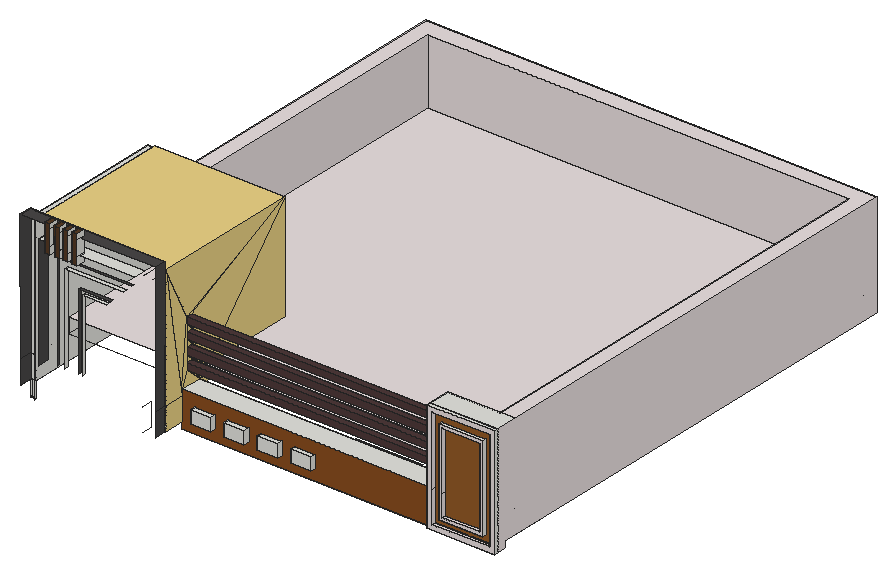
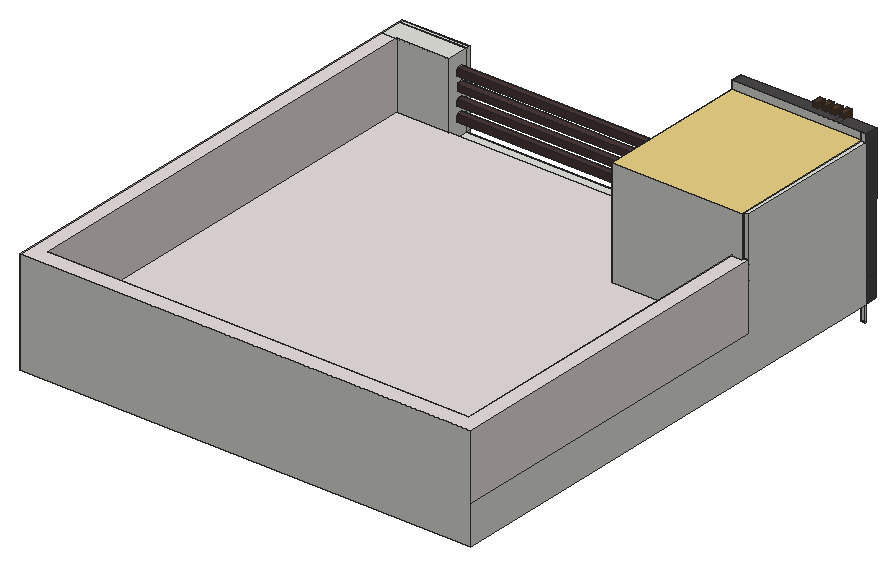
# SketchUp Ruby script. Lengths in inches.
U = 1.inch
M = Sketchup.active_model
def pt(a) = Geom::Point3d.new(a.map { |v| v * U })
def face(e, loops, mat)
  f = e.add_face(loops[0].map { |a| pt(a) })
  loops[1..].each { |l| e.add_face(l.map { |a| pt(a) }).erase! }
  f.material = f.back_material = mat if mat
  f
end
# faces: each face lists its corners as indices into pts; further lists are holes
def faces(e, pts, list, mat = nil) = list.each { |f| face(e, (f[0].is_a?(Array) ? f : [f]).map { |l| l.map { |i| pts[i] } }, mat) }
# xy, xz, yz: faces in a plane at the given z, y or x. An outline is a flat list of corners, or four numbers for a rectangle; further outlines are holes
def ring(l) = l.size == 4 ? [[l[0], l[1]], [l[2], l[1]], [l[2], l[3]], [l[0], l[3]]] : l.each_slice(2).to_a
def flat(e, list, mat, &to3) = list.each { |f| face(e, (f[0].is_a?(Array) ? f : [f]).map { |l| ring(l).map { |u, v| to3.(u, v) } }, mat) }
def xy(e, z, list, mat = nil) = flat(e, list, mat) { |x, y| [x, y, z] }
def xz(e, y, list, mat = nil) = flat(e, list, mat) { |x, z| [x, y, z] }
def yz(e, x, list, mat = nil) = flat(e, list, mat) { |y, z| [x, y, z] }
def lines(e, pts, list) = list.each { |a, b| e.add_line(pt(pts[a]), pt(pts[b])) }
# prism: a flat outline (further loops are holes) pulled along v
def prism(e, loops, v, mat = nil)
  f = face(e, loops, mat); d = Geom::Vector3d.new(v.map { |x| x * U })
  f.pushpull(f.normal.samedirection?(d) ? d.length : -d.length)
end
def box(e, o, s, mat = nil) = prism(e, [[o, [o[0] + s[0], o[1], o[2]], [o[0] + s[0], o[1] + s[1], o[2]], [o[0], o[1] + s[1], o[2]]]], [0, 0, s[2]], mat)
def at(x, y, z, deg = 0) = Geom::Transformation.translation(pt([x, y, z])) * Geom::Transformation.rotation(ORIGIN, Z_AXIS, deg.degrees)
def axes(o, x, y, z) = Geom::Transformation.new([*x, 0, *y, 0, *z, 0, *pt(o).to_a, 1])
def part(name) = M.definitions.add(name)
# library, detail: a bought-in or finely detailed component or shape, given as its bounding box
def library(name, o, s) = part(name).tap { |d| box(d.entities, o, s) }
def detail(e, o, s) = box(e.add_group.entities, o, s)
def put(e, d, t, mat = nil) = e.add_instance(d, t).tap { |i| i.material = mat if mat }
def group(e, t, mat = nil) = e.add_group.tap { |g| g.transformation = t; g.material = mat if mat }.entities
root = M.entities
M.materials.add("Generic").color = [136, 77, 32]
M.materials.add("Generic\#1").color = [73, 71, 71]
M.materials.add("Generic\#2").color = [78, 57, 57]
M.materials.add("Generic\#3").color = [235, 210, 133]
M.materials.add("Generic\#4").color = [84, 58, 36]
M.materials.add("Generic\#5").color = [232, 222, 222]
M.materials.add("Material \#1").color = [140, 140, 140]
M.materials.add("[Wood Floor Parquet]").color = [145, 89, 39]
xy(root,225.757,[[371.53,115.15,371.464,115.17,371.474,115.185],[371.53,115.15,371.474,115.185,371.533,115.167],[371.53,115.15,371.533,115.167,371.6,115.15],[371.6,115.15,371.533,115.167,371.597,115.167],[371.6,115.15,371.597,115.167,371.667,115.17],
  [371.597,115.167,371.657,115.185,371.667,115.17],[371.464,115.17,371.41,115.209,371.425,115.22],[371.464,115.17,371.425,115.22,371.474,115.185],[371.667,115.17,371.657,115.185,371.721,115.209],[371.657,115.185,371.705,115.22,371.721,115.209],
  [371.41,115.209,371.374,115.261,371.393,115.267],[371.41,115.209,371.393,115.267,371.425,115.22],[371.721,115.209,371.705,115.22,371.756,115.261],[371.705,115.22,371.737,115.267,371.756,115.261],[371.374,115.261,371.362,115.32,371.382,115.32],
  [371.374,115.261,371.382,115.32,371.393,115.267],[371.756,115.261,371.737,115.267,371.768,115.32],[371.737,115.267,371.748,115.32,371.768,115.32],[371.362,115.32,371.374,115.379,371.393,115.373],[371.362,115.32,371.393,115.373,371.382,115.32],
  [371.748,115.32,371.737,115.373,371.756,115.379],[371.748,115.32,371.756,115.379,371.768,115.32],[371.393,115.373,371.374,115.379,371.425,115.42],[371.737,115.373,371.705,115.42,371.721,115.431],[371.737,115.373,371.721,115.431,371.756,115.379],
  [371.374,115.379,371.41,115.431,371.425,115.42],[371.425,115.42,371.41,115.431,371.474,115.454],[371.705,115.42,371.657,115.454,371.667,115.469],[371.705,115.42,371.667,115.469,371.721,115.431],[371.41,115.431,371.464,115.469,371.474,115.454],
  [371.474,115.454,371.464,115.469,371.533,115.473],[371.657,115.454,371.597,115.473,371.6,115.49],[371.657,115.454,371.6,115.49,371.667,115.469],[371.464,115.469,371.53,115.49,371.533,115.473],[371.533,115.473,371.53,115.49,371.597,115.473],
  [371.597,115.473,371.53,115.49,371.6,115.49]],"Material \#1")
xy(root,225.773,[[371.53,115.15,371.533,115.167,371.464,115.17],[371.53,115.15,371.597,115.167,371.533,115.167],[371.53,115.15,371.6,115.15,371.597,115.167],[371.6,115.15,371.657,115.185,371.597,115.167],[371.6,115.15,371.667,115.17,371.657,115.185],
  [371.533,115.167,371.474,115.185,371.464,115.17],[371.464,115.17,371.474,115.185,371.41,115.209],[371.667,115.17,371.705,115.22,371.657,115.185],[371.667,115.17,371.721,115.209,371.705,115.22],[371.474,115.185,371.425,115.22,371.41,115.209],
  [371.41,115.209,371.425,115.22,371.374,115.261],[371.721,115.209,371.737,115.267,371.705,115.22],[371.721,115.209,371.756,115.261,371.737,115.267],[371.425,115.22,371.393,115.267,371.374,115.261],[371.374,115.261,371.393,115.267,371.362,115.32],
  [371.756,115.261,371.748,115.32,371.737,115.267],[371.756,115.261,371.768,115.32,371.748,115.32],[371.393,115.267,371.382,115.32,371.362,115.32],[371.362,115.32,371.382,115.32,371.374,115.379],[371.382,115.32,371.393,115.373,371.374,115.379],
  [371.748,115.32,371.768,115.32,371.737,115.373],[371.768,115.32,371.756,115.379,371.737,115.373],[371.393,115.373,371.41,115.431,371.374,115.379],[371.393,115.373,371.425,115.42,371.41,115.431],[371.737,115.373,371.756,115.379,371.705,115.42],
  [371.756,115.379,371.721,115.431,371.705,115.42],[371.425,115.42,371.464,115.469,371.41,115.431],[371.425,115.42,371.474,115.454,371.464,115.469],[371.705,115.42,371.721,115.431,371.657,115.454],[371.721,115.431,371.667,115.469,371.657,115.454],
  [371.474,115.454,371.53,115.49,371.464,115.469],[371.474,115.454,371.533,115.473,371.53,115.49],[371.657,115.454,371.667,115.469,371.597,115.473],[371.667,115.469,371.6,115.49,371.597,115.473],[371.533,115.473,371.6,115.49,371.53,115.49],
  [371.533,115.473,371.597,115.473,371.6,115.49]],"Material \#1")
xy(root,227.533,[[205.199,114.8125,268.449,169.8125]])
xy(root,229.316,[[371.53,115.15,371.464,115.17,371.533,115.167],[371.53,115.15,371.533,115.167,371.597,115.167],[371.53,115.15,371.597,115.167,371.6,115.15],[371.6,115.15,371.597,115.167,371.657,115.185],[371.6,115.15,371.657,115.185,371.667,115.17],
  [371.533,115.167,371.464,115.17,371.474,115.185],[371.464,115.17,371.41,115.209,371.474,115.185],[371.667,115.17,371.657,115.185,371.705,115.22],[371.667,115.17,371.705,115.22,371.721,115.209],[371.474,115.185,371.41,115.209,371.425,115.22],
  [371.41,115.209,371.374,115.261,371.425,115.22],[371.721,115.209,371.705,115.22,371.737,115.267],[371.721,115.209,371.737,115.267,371.756,115.261],[371.425,115.22,371.374,115.261,371.393,115.267],[371.374,115.261,371.362,115.32,371.393,115.267],
  [371.756,115.261,371.737,115.267,371.748,115.32],[371.756,115.261,371.748,115.32,371.768,115.32],[371.393,115.267,371.362,115.32,371.382,115.32],[371.362,115.32,371.374,115.379,371.382,115.32],[371.382,115.32,371.374,115.379,371.393,115.373],
  [371.748,115.32,371.737,115.373,371.768,115.32],[371.768,115.32,371.737,115.373,371.756,115.379],[371.393,115.373,371.374,115.379,371.41,115.431],[371.393,115.373,371.41,115.431,371.425,115.42],[371.737,115.373,371.705,115.42,371.756,115.379],
  [371.756,115.379,371.705,115.42,371.721,115.431],[371.425,115.42,371.41,115.431,371.464,115.469],[371.425,115.42,371.464,115.469,371.474,115.454],[371.705,115.42,371.657,115.454,371.721,115.431],[371.721,115.431,371.657,115.454,371.667,115.469],
  [371.474,115.454,371.464,115.469,371.53,115.49],[371.474,115.454,371.53,115.49,371.533,115.473],[371.657,115.454,371.597,115.473,371.667,115.469],[371.667,115.469,371.597,115.473,371.6,115.49],[371.533,115.473,371.53,115.49,371.6,115.49],
  [371.533,115.473,371.6,115.49,371.597,115.473]],"Material \#1")
xy(root,229.332,[[371.53,115.15,371.474,115.185,371.464,115.17],[371.53,115.15,371.533,115.167,371.474,115.185],[371.53,115.15,371.6,115.15,371.533,115.167],[371.6,115.15,371.597,115.167,371.533,115.167],[371.6,115.15,371.667,115.17,371.597,115.167],
  [371.597,115.167,371.667,115.17,371.657,115.185],[371.464,115.17,371.425,115.22,371.41,115.209],[371.464,115.17,371.474,115.185,371.425,115.22],[371.667,115.17,371.721,115.209,371.657,115.185],[371.657,115.185,371.721,115.209,371.705,115.22],
  [371.41,115.209,371.393,115.267,371.374,115.261],[371.41,115.209,371.425,115.22,371.393,115.267],[371.721,115.209,371.756,115.261,371.705,115.22],[371.705,115.22,371.756,115.261,371.737,115.267],[371.374,115.261,371.382,115.32,371.362,115.32],
  [371.374,115.261,371.393,115.267,371.382,115.32],[371.756,115.261,371.768,115.32,371.737,115.267],[371.737,115.267,371.768,115.32,371.748,115.32],[371.362,115.32,371.382,115.32,371.393,115.373],[371.362,115.32,371.393,115.373,371.374,115.379],
  [371.748,115.32,371.756,115.379,371.737,115.373],[371.748,115.32,371.768,115.32,371.756,115.379],[371.393,115.373,371.425,115.42,371.374,115.379],[371.737,115.373,371.721,115.431,371.705,115.42],[371.737,115.373,371.756,115.379,371.721,115.431],
  [371.374,115.379,371.425,115.42,371.41,115.431],[371.425,115.42,371.474,115.454,371.41,115.431],[371.705,115.42,371.667,115.469,371.657,115.454],[371.705,115.42,371.721,115.431,371.667,115.469],[371.41,115.431,371.474,115.454,371.464,115.469],
  [371.474,115.454,371.533,115.473,371.464,115.469],[371.657,115.454,371.6,115.49,371.597,115.473],[371.657,115.454,371.667,115.469,371.6,115.49],[371.464,115.469,371.533,115.473,371.53,115.49],[371.533,115.473,371.597,115.473,371.53,115.49],
  [371.597,115.473,371.6,115.49,371.53,115.49]],"Material \#1")
xy(root,235.716,[[330.35,114.8125,374.475,141.3125]])
xy(root,255.6875,[[361.519,58.125,424.885,61.6875],[127.575,61.6875,402.977,70.125],[402.977,61.6875,412.79,70.125],[412.79,61.6875,419.477,70.125],[419.477,61.6875,424.885,70.125]])
xy(root,260.286,[[366.118,58.125,420.286,61.6875]],"Generic\#5")
xy(root,261.937,[[0.012,30.0625,0.509,42.5]])
xy(root,261.9375,[[4.322,41.4375,4.387,42.5],[4.387,41.4375,4.884,42.5],[4.322,42.5,4.884,42.5,4.885,114.8125,4.322,114.8125],[412.79,70.125,419.477,79.528]])
xy(root,261.9375,[[127.575,70.125,127.575,114.8125,424.885,114.8125,424.885,70.125,419.477,70.125,419.477,79.528,412.79,79.528,412.79,70.125]],"Generic\#3")
xy(root,266.347,[[139.227,56.9375,158.441,61.6875],[170.664,56.9375,189.878,61.6875],[202.102,56.9375,221.316,61.6875],[233.539,56.9375,252.753,61.6875]])
xy(root,266.989,[[372.821,58.125,413.583,61.6875]],"Generic\#5")
xy(root,269.637,[[375.469,58.125,410.935,61.6875]],"Generic\#5")
xy(root,278.222,[[139.227,56.9375,158.441,61.6875],[170.664,56.9375,189.878,61.6875],[202.102,56.9375,221.316,61.6875],[233.539,56.9375,252.753,61.6875]])
xy(root,289.375,[[127.57,61.6875,361.519,82.1875]])
xy(root,298,[[4.322,82.1875,411.072,82.1875,411.072,493.0625,14.375,493.0625,14.375,180.616,4.322,180.616]],"Generic\#5")
xy(root,345.113,[[375.469,58.125,410.935,61.6875]],"Generic\#5")
xy(root,347.761,[[372.821,58.125,413.583,61.6875]])
xy(root,351.982,[[51.311,39.25,73.882,42.5]])
xy(root,355.589,[[366.118,58.125,420.286,61.6875]],"Generic\#5")
xy(root,355.683,[[47.609,39.25,77.584,42.5]],"Generic\#1")
xy(root,360.1875,[[361.519,58.125,424.885,61.6875],[361.519,61.6875,424.885,82.1875]])
xy(root,360.1875,[[411.072,82.1875,424.885,82.1875,424.885,508.6875,0,508.6875,0,180.616,14.375,180.616,14.375,493.0625,411.072,493.0625]],"Generic\#5")
xy(root,368.38,[[34.912,39.25,90.279,42.5]])
xy(root,375.663,[[27.628,39.25,97.5625,41.4375]],"Generic\#1")
xy(root,384.421,[[26.151,26.375,31.026,41.4375],[35.089,26.375,39.964,34.4375],[43.339,26.375,48.214,34.4375],[51.589,26.375,56.464,34.4375]],"Generic\#4")
xy(root,391.47,[[17.071,30.0625,26.151,41.4375],[31.026,30.0625,108.119,41.4375]])
xy(root,398.914,[[0,42.5,4.322,180.616]])
xy(root,406.289,[[0,30.0625,26.108,30.0625,26.108,41.4375,4.322,41.4375,4.322,42.5,0,42.5],[26.108,34.4375,30.983,41.4375]],"Generic\#1")
xy(root,410.825,[[26.095,26.375,30.97,34.4375],[35.033,26.375,39.908,34.4375],[43.283,26.375,48.158,34.4375],[51.533,26.375,56.408,34.4375]],"Generic\#4")
xz(root,26.375,[[26.151,384.421,31.026,384.421,31.026,391.47,30.983,406.289,30.97,410.825,26.095,410.825,26.151,391.47],[35.089,384.421,39.964,384.421,39.964,391.47,39.921,406.289,39.908,410.825,35.033,410.825,35.089,391.47],[43.339,384.421,48.214,384.421,48.214,391.47,48.171,406.289,48.158,410.825,43.283,410.825,43.339,391.47],[51.589,384.421,56.464,384.421,56.464,391.47,56.421,406.289,56.408,410.825,51.533,410.825,51.589,391.47]],"Generic\#4")
xz(root,34.4375,[[35.089,384.421,35.089,391.47,35.033,410.825,39.908,410.825,39.921,406.289,39.964,391.47,39.964,384.421],[43.339,384.421,43.339,391.47,43.283,410.825,48.158,410.825,48.171,406.289,48.214,391.47,48.214,384.421],[51.589,384.421,51.589,391.47,51.533,410.825,56.408,410.825,56.421,406.289,56.464,391.47,56.464,384.421],[26.108,406.289,26.095,410.825,30.97,410.825,30.983,406.289]],"Generic\#4")
xz(root,41.4375,[[26.151,384.421,31.026,391.47],[4.322,398.914,4.375,406.289],[4.375,398.914,4.375,406.289,30.983,406.289,127.563,406.29,127.563,398.915]])
xz(root,42.5,[[0.001,246.511,0.51,247.422],[0.51,246.511,4.885,247.422],[0.001,247.422,0.51,247.422,0.509,261.937,0.012,261.937,0,261.9375],[0.51,247.422,4.885,247.422,4.884,261.9375,3.682,261.9375,0.509,261.937],[0.012,261.937,0.008,283.875,0,398.914,0,261.9375],
  [0.012,261.937,0.509,261.937,3.682,261.9375,4.322,261.9375,4.322,283.875,0.008,283.875],[0.008,283.875,4.322,283.875,4.322,398.914,0,398.914],[0,398.914,4.322,406.289]])
xz(root,56.9375,[[139.227,266.347,158.441,278.222],[170.664,266.347,189.878,278.222],[202.102,266.347,221.316,278.222],[233.539,266.347,252.753,278.222]])
xz(root,58.125,[[[361.519,255.6875,424.885,360.1875],[366.118,260.286,420.286,355.589]],[[372.821,266.989,413.583,347.761],[375.469,269.637,410.935,345.113]]],"Generic\#5")
xz(root,61.6875,[[[361.519,255.6875,424.885,360.1875],[366.118,260.286,420.286,355.589]]])
xz(root,61.6875,[[[127.575,255.6875,361.519,255.6875,361.519,289.375,127.57,289.375,127.57,283.875,127.575,261.9375],[233.539,266.347,252.753,278.222],[202.102,266.347,221.316,278.222],[170.664,266.347,189.878,278.222],[139.227,266.347,158.441,278.222]]],"Generic")
xz(root,61.6875,[[[366.118,260.286,420.286,355.589],[372.821,266.989,413.583,347.761]],[375.469,269.637,410.935,345.113]],"[Wood Floor Parquet]")
xz(root,67,[[361.518,316.263,361.519,316.263,361.519,322.513]])
xz(root,67,[[127.568,303.307,361.519,303.322,361.519,303.5625,361.518,309.572,127.568,309.557],[127.568,316.247,361.518,316.263,361.519,322.513,127.568,322.497],[127.568,329.1875,361.52,329.203,361.519,335.453,127.568,335.4375],[127.568,342.128,361.395,342.143,361.394,348.393,127.568,348.378]],"Generic\#2")
xz(root,70.125,[[127.575,255.6875,402.977,261.9375],[402.977,255.6875,412.79,261.9375],[412.79,255.6875,419.477,261.9375],[419.477,255.6875,424.885,261.9375]])
xz(root,73.25,[[361.518,316.263,361.519,322.513,361.519,316.263]])
xz(root,73.25,[[127.568,303.307,127.568,309.557,361.518,309.572,361.519,303.5625,361.519,303.322],[127.568,316.247,127.568,322.497,361.519,322.513,361.518,316.263],[127.568,329.1875,127.568,335.4375,361.519,335.453,361.52,329.203],[127.568,342.128,127.568,348.378,361.394,348.393,361.395,342.143]],"Generic\#2")
xz(root,81.25,[[116.45,261.937,118.45,261.9375,118.445,283.875,116.445,283.875]])
xz(root,82.1875,[[127.57,283.875,361.519,289.375],[361.519,298,411.072,360.1875]])
xz(root,180.616,[[0,360.1875,4.322,398.914]])
xz(root,180.616,[[0,298,4.322,360.1875],[4.322,298,14.375,360.1875]],"Generic\#5")
xz(root,183.125,[[4.383,283.875,4.375,398.914,127.563,398.915,127.57,283.875]])
xz(root,493.0625,[[14.375,298,411.072,360.1875]],"Generic\#5")
xz(root,508.6875,[[0,261.9375,424.885,360.1875]])
yz(root,0,[[42.5,261.9375,42.5,398.914,180.616,398.914,180.616,298,508.6875,298,508.6875,261.9375]])
yz(root,0,[[180.616,298,508.6875,360.1875]],"Generic\#5")
yz(root,4.322,[[41.4375,261.9375,42.5,283.875],[42.5,261.9375,493.6875,261.9375,493.6875,283.875,82.1875,283.875,82.1875,298,180.616,298,180.616,398.914,42.5,398.914],[41.4375,283.875,42.5,406.289]])
yz(root,4.885,[[41.4375,246.511,42.5,247.422]])
yz(root,14.375,[[180.616,298,493.0625,360.1875]],"Generic\#5")
yz(root,26.151,[[26.375,384.421,41.4375,391.47]],"Generic\#4")
yz(root,31.026,[[26.375,384.421,41.4375,391.47]])
yz(root,35.089,[[26.375,384.421,34.4375,391.47]],"Generic\#4")
yz(root,39.964,[[26.375,384.421,34.4375,391.47]])
yz(root,43.339,[[26.375,384.421,34.4375,391.47]],"Generic\#4")
yz(root,48.214,[[26.375,384.421,34.4375,391.47]])
yz(root,51.589,[[26.375,384.421,34.4375,391.47]],"Generic\#4")
yz(root,56.464,[[26.375,384.421,34.4375,391.47]])
yz(root,127.568,[[67,309.557,73.25,309.557,67,316.247],[73.25,309.557,73.25,316.247,67,316.247],[67,322.497,73.25,322.497,67,329.1875],[73.25,322.497,73.25,329.1875,67,329.1875],[67,335.4375,73.25,335.4375,67,342.128],
  [73.25,335.4375,73.25,342.128,67,342.128]],"Generic\#3")
yz(root,127.57,[[82.1875,283.875,183.125,283.875,82.1875,289.375]],"Generic\#3")
yz(root,139.227,[[56.9375,266.347,61.6875,278.222]])
yz(root,158.441,[[56.9375,266.347,61.6875,278.222]])
yz(root,170.664,[[56.9375,266.347,61.6875,278.222]])
yz(root,189.878,[[56.9375,266.347,61.6875,278.222]])
yz(root,202.102,[[56.9375,266.347,61.6875,278.222]])
yz(root,221.316,[[56.9375,266.347,61.6875,278.222]])
yz(root,233.539,[[56.9375,266.347,61.6875,278.222]])
yz(root,252.753,[[56.9375,266.347,61.6875,278.222]])
yz(root,361.519,[[58.125,255.6875,61.6875,289.375],[58.125,289.375,61.6875,360.1875],[61.6875,289.375,82.1875,360.1875],[67,316.263,73.25,322.513]])
yz(root,366.118,[[58.125,260.286,61.6875,289.375],[58.125,289.375,61.6875,355.589]],"Generic\#5")
yz(root,372.821,[[58.125,289.375,61.6875,347.761]])
yz(root,372.821,[[58.125,266.989,61.6875,289.375]],"Generic\#5")
yz(root,375.469,[[58.125,269.637,61.6875,289.375],[58.125,289.375,61.6875,345.113]],"Generic\#5")
yz(root,410.935,[[58.125,269.637,61.6875,345.113]],"Generic\#5")
yz(root,411.072,[[82.1875,298,493.0625,360.1875]],"Generic\#5")
yz(root,413.583,[[58.125,266.989,61.6875,347.761]])
yz(root,420.286,[[58.125,260.286,61.6875,355.589]],"Generic\#5")
yz(root,424.885,[[58.125,255.6875,61.6875,360.1875]])
yz(root,424.885,[[61.6875,255.6875,70.125,255.6875,70.125,261.9375,508.6875,261.9375,508.6875,360.1875,61.6875,360.1875]],"Generic\#5")
p = [[4.884,42.5,261.9375],[4.885,42.5,247.422],[4.885,41.4375,247.422],[4.884,41.4375,261.9375],[0.008,42.5,283.875],[0.012,42.5,261.937],
  [0.012,30.0625,261.937],[0.008,30.0625,283.875],[127.575,30.0625,261.9375],[127.575,41.4375,261.9375],[127.57,41.4375,283.875],[127.57,30.0625,283.875],
  [127.575,42.5,261.9375],[127.57,42.5,283.875],[127.57,61.6875,283.875],[127.575,61.6875,261.9375],[0,42.5,398.914],[0,30.0625,406.289],
  [0,42.5,406.289],[17.077,30.0625,283.877],[17.077,41.4375,283.877],[17.071,41.4375,391.47],[17.071,30.0625,391.47],[127.563,41.4375,398.915],
  [127.563,41.4375,406.29],[127.563,30.0625,406.29],[27.628,39.25,375.663],[27.628,41.4375,375.663],[27.634,41.4375,283.878],[27.634,39.25,283.878],
  [34.917,42.5,283.879],[34.912,42.5,368.38],[34.912,39.25,368.38],[34.917,39.25,283.879],[47.609,42.5,355.683],[47.614,42.5,283.881],
  [47.614,39.25,283.881],[47.609,39.25,355.683],[51.316,42.5,283.882],[51.311,42.5,351.982],[51.311,39.25,351.982],[51.316,39.25,283.882],
  [127.563,42.5,398.915],[127.57,61.6875,289.375],[127.57,183.125,283.875],[127.563,183.125,398.915],[127.57,82.1875,289.375],[127.568,67,348.378],
  [127.568,67,303.307],[127.568,67,309.557],[127.568,67,316.247],[127.568,67,322.497],[127.568,67,329.1875],[127.568,67,335.4375],
  [127.568,67,342.128],[127.568,73.25,303.307],[127.568,73.25,309.557],[127.568,73.25,316.247],[127.568,73.25,322.497],[127.568,73.25,329.1875],
  [127.568,73.25,335.4375],[127.568,73.25,342.128],[127.568,73.25,348.378],[361.519,73.25,303.322],[361.519,67,303.322],[361.518,67,309.572],
  [361.519,67,303.5625],[361.519,73.25,303.5625],[361.518,73.25,309.572],[361.518,73.25,316.263],[361.519,73.25,316.263],[361.519,67,316.263],
  [361.518,67,316.263],[361.519,67,322.513],[361.519,73.25,322.513],[361.52,73.25,329.203],[361.52,67,329.203],[361.519,67,335.453],
  [361.519,73.25,335.453],[361.395,73.25,342.143],[361.395,67,342.143],[361.394,67,348.393],[361.394,73.25,348.393],[26.151,30.0625,391.47],
  [26.151,26.375,391.47],[26.095,26.375,410.825],[26.095,34.4375,410.825],[26.108,34.4375,406.289],[26.108,30.0625,406.289],[31.026,30.0625,391.47],
  [30.983,30.0625,406.289],[30.983,26.375,406.289],[31.026,26.375,391.47],[35.089,26.375,391.47],[35.033,26.375,410.825],[35.033,34.4375,410.825],
  [35.089,34.4375,391.47],[35.089,30.0625,391.47],[39.921,26.375,406.289],[39.964,26.375,391.47],[39.964,30.0625,391.47],[39.964,34.4375,391.47],
  [39.921,34.4375,406.289],[39.921,30.0625,406.289],[43.339,26.375,391.47],[43.283,26.375,410.825],[43.283,34.4375,410.825],[43.339,34.4375,391.47],
  [43.339,30.0625,391.47],[48.171,26.375,406.289],[48.214,26.375,391.47],[48.214,30.0625,391.47],[48.214,34.4375,391.47],[48.171,34.4375,406.289],
  [48.171,30.0625,406.289],[51.589,26.375,391.47],[51.533,26.375,410.825],[51.533,34.4375,410.825],[51.589,34.4375,391.47],[51.589,30.0625,391.47],
  [56.421,26.375,406.289],[56.464,26.375,391.47],[56.464,30.0625,391.47],[56.464,34.4375,391.47],[56.421,34.4375,406.289],[56.421,30.0625,406.289],
  [4.375,183.125,398.914],[4.375,41.4375,398.914],[30.97,34.4375,410.825],[30.97,26.375,410.825],[30.983,34.4375,406.289],[39.908,26.375,410.825],
  [39.908,34.4375,410.825],[48.158,26.375,410.825],[48.158,34.4375,410.825],[56.408,26.375,410.825],[56.408,34.4375,410.825],[30.983,41.4375,406.289],
  [424.885,493.6875,283.875],[4.322,493.6875,283.875],[4.322,61.6875,283.875],[4.383,61.6875,283.875],[412.79,79.528,262.375],[412.79,70.125,262.375],
  [412.79,70.125,261.9375],[15.188,42.5,389.977],[15.188,81.25,389.977],[17.071,42.5,386.22],[17.071,105.25,386.22],[114.869,78.523,386.22],
  [114.869,105.25,386.22],[105.994,42.5,386.219],[105.994,78.523,386.219],[114.869,42.5,386.22],[424.885,82.1875,283.875],[361.519,82.1875,283.875],
  [127.57,82.1875,283.875],[4.322,82.1875,283.875],[114.88,41.4375,261.936],[114.876,41.4375,283.873],[114.876,30.0625,283.873],[114.88,30.0625,261.936]]
faces(root,p,[[0,1,2,3],[12,13,10,9],[30,31,32,33],[38,39,40,41],[48,55,63,64],[65,66,64,63,67,68],[50,57,69,70,71,72],[52,59,75,76],
  [77,76,75,78],[54,61,79,80],[81,80,79,82],[89,90,91,92],[98,99,100,101,102,103],[109,110,111,112,113,114],[120,121,122,123,124,125],[128,129,91,90,130],
  [131,98,103,102,132],[133,109,114,113,134],[135,120,125,124,136]])
faces(root,p,[[4,5,6,7],[8,9,10,11],[16,4,7,17,18],[19,20,21,22],[11,10,23,24,25],[26,27,28,29],[34,35,36,37],[24,137,130,90,103,114,125,25]],"Generic\#1")
faces(root,p,[[14,13,12,15],[13,42,23,10],[43,42,14],[14,42,13],[44,45,46],[47,42,43],[43,46,48],[48,49,50,51,52,53,54,47,43],
  [55,48,46],[56,55,46],[57,56,46],[58,57,46],[59,58,46],[60,59,46],[61,60,46],[62,61,46],
  [46,45,62],[45,42,47],[62,45,47],[126,127,23,42,45]],"Generic\#3")
faces(root,p,[[56,49,65,68],[58,51,73,74],[60,53,77,78],[62,47,81,82]],"Generic\#2")
faces(root,p,[[83,84,85,86,87,88],[93,94,95,96,97],[104,105,106,107,108],[115,116,117,118,119]],"Generic\#4")
lines(root,p,[[138,139],[140,141],[142,143],[144,143],[145,146],[147,148],[149,150],[151,152],[153,149],[154,155],[156,157],[158,159],
  [159,160],[158,161]])
